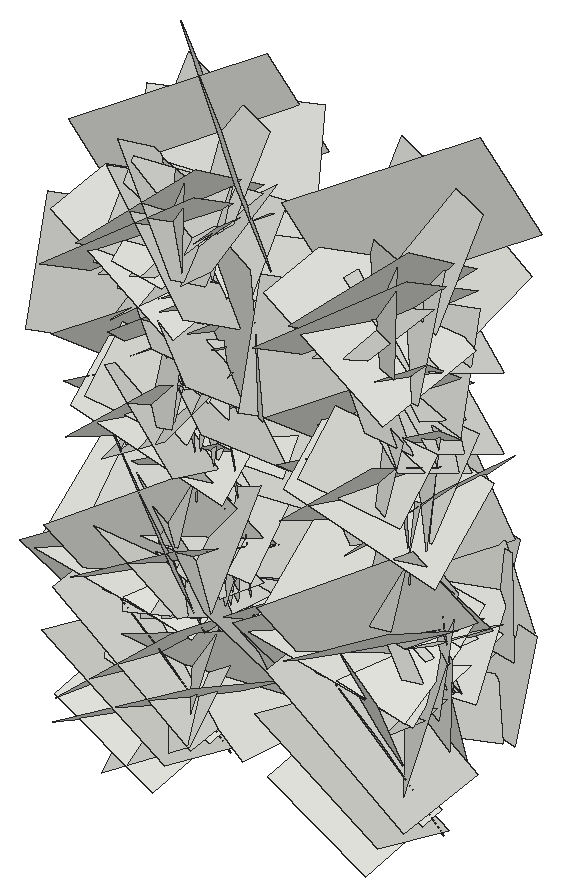
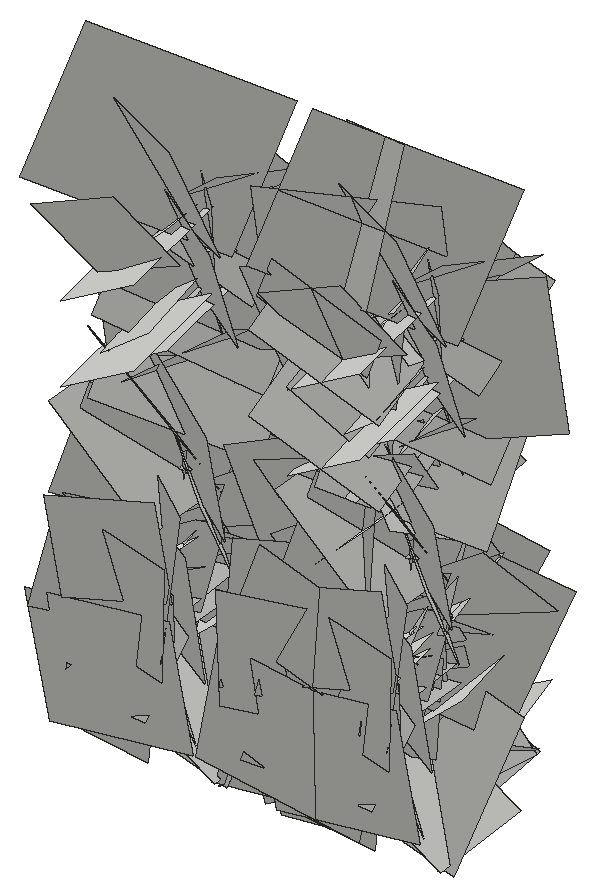
# SketchUp Ruby script. Lengths in inches.
U = 1.inch
M = Sketchup.active_model
def pt(a) = Geom::Point3d.new(a.map { |v| v * U })
def face(e, loops, mat)
  f = e.add_face(loops[0].map { |a| pt(a) })
  loops[1..].each { |l| e.add_face(l.map { |a| pt(a) }).erase! }
  f.material = f.back_material = mat if mat
  f
end
# faces: each face lists its corners as indices into pts; further lists are holes
def faces(e, pts, list, mat = nil) = list.each { |f| face(e, (f[0].is_a?(Array) ? f : [f]).map { |l| l.map { |i| pts[i] } }, mat) }
# xy, xz, yz: faces in a plane at the given z, y or x. An outline is a flat list of corners, or four numbers for a rectangle; further outlines are holes
def ring(l) = l.size == 4 ? [[l[0], l[1]], [l[2], l[1]], [l[2], l[3]], [l[0], l[3]]] : l.each_slice(2).to_a
def flat(e, list, mat, &to3) = list.each { |f| face(e, (f[0].is_a?(Array) ? f : [f]).map { |l| ring(l).map { |u, v| to3.(u, v) } }, mat) }
def xy(e, z, list, mat = nil) = flat(e, list, mat) { |x, y| [x, y, z] }
def xz(e, y, list, mat = nil) = flat(e, list, mat) { |x, z| [x, y, z] }
def yz(e, x, list, mat = nil) = flat(e, list, mat) { |y, z| [x, y, z] }
def lines(e, pts, list) = list.each { |a, b| e.add_line(pt(pts[a]), pt(pts[b])) }
# prism: a flat outline (further loops are holes) pulled along v
def prism(e, loops, v, mat = nil)
  f = face(e, loops, mat); d = Geom::Vector3d.new(v.map { |x| x * U })
  f.pushpull(f.normal.samedirection?(d) ? d.length : -d.length)
end
def box(e, o, s, mat = nil) = prism(e, [[o, [o[0] + s[0], o[1], o[2]], [o[0] + s[0], o[1] + s[1], o[2]], [o[0], o[1] + s[1], o[2]]]], [0, 0, s[2]], mat)
def at(x, y, z, deg = 0) = Geom::Transformation.translation(pt([x, y, z])) * Geom::Transformation.rotation(ORIGIN, Z_AXIS, deg.degrees)
def axes(o, x, y, z) = Geom::Transformation.new([*x, 0, *y, 0, *z, 0, *pt(o).to_a, 1])
def part(name) = M.definitions.add(name)
# library, detail: a bought-in or finely detailed component or shape, given as its bounding box
def library(name, o, s) = part(name).tap { |d| box(d.entities, o, s) }
def detail(e, o, s) = box(e.add_group.entities, o, s)
def put(e, d, t, mat = nil) = e.add_instance(d, t).tap { |i| i.material = mat if mat }
def group(e, t, mat = nil) = e.add_group.tap { |g| g.transformation = t; g.material = mat if mat }.entities
root = M.entities
c1 = part("Component\#6")
p = [[0.01,0,0],[0,3.24,4.54],[4.32,3.24,4.54],[4.33,0,0]]
faces(c1.entities,p,[[0,1,2,3]])
put(root,c1,axes([410.71,208.64,6.82],[0.0498,0.28937,-0.67344],[0.06797,-0.67386,-0.28508],[0.77398,0.04056,0.06836]))
put(root,c1,axes([404.88,210.125,0.49],[-0.19083,-0.77607,-0.35788],[-0.04853,-0.35645,0.796],[-0.90459,0.18284,0.03279]))
put(root,c1,axes([400.91,210.125,0.49],[0.19083,-0.77607,-0.35788],[0.04853,-0.35645,0.796],[0.90459,0.18284,0.03279]))
put(root,c1,axes([414.68,210.125,0.49],[-0.19083,-0.77607,-0.35788],[-0.04853,-0.35645,0.796],[-0.90459,0.18284,0.03279]))
put(root,c1,axes([404.88,210.53,-0.53],[0.13793,-1.11303,0.36033],[-0.12678,0.348,1.11812],[-1.23359,-0.16021,-0.07463]))
put(root,c1,axes([400.91,210.53,-0.53],[-0.13793,-1.11303,0.36033],[0.12678,0.348,1.11812],[1.23359,-0.16021,-0.07463]))
put(root,c1,axes([414.68,210.53,-0.53],[0.13793,-1.11303,0.36033],[-0.12678,0.348,1.11812],[-1.23359,-0.16021,-0.07463]))
put(root,c1,axes([404.88,209.89,15.21],[-0.14915,-0.31655,-0.61374],[-0.00846,-0.62556,0.32448],[-0.73195,0.07174,0.12131]))
put(root,c1,axes([400.91,209.89,15.21],[0.14915,-0.31655,-0.61374],[0.00846,-0.62556,0.32448],[0.73195,0.07174,0.12131]))
put(root,c1,axes([414.68,209.89,15.21],[-0.14915,-0.31655,-0.61374],[-0.00846,-0.62556,0.32448],[-0.73195,0.07174,0.12131]))
put(root,c1,axes([400.91,209.73,11.28],[-0.10776,-0.78869,0.28769],[-0.10217,0.29884,0.7852],[0.88401,-0.0616,0.12582]))
put(root,c1,axes([404.88,209.73,11.28],[0.10776,-0.78869,0.28769],[0.10217,0.29884,0.7852],[-0.88401,-0.0616,0.12582]))
put(root,c1,axes([410.71,209.73,11.28],[-0.10776,-0.78869,0.28769],[-0.10217,0.29884,0.7852],[0.88401,-0.0616,0.12582]))
put(root,c1,axes([404.88,208.44,11.85],[0.18719,0.63062,-0.8853],[0.07209,-0.90156,-0.62864],[-1.1499,0.04614,-0.18352]))
put(root,c1,axes([414.68,208.44,11.85],[0.18719,0.63062,-0.8853],[0.07209,-0.90156,-0.62864],[-1.1499,0.04614,-0.18352]))
put(root,c1,axes([400.91,208.44,11.85],[-0.18719,0.63062,-0.8853],[-0.07209,-0.90156,-0.62864],[1.1499,0.04614,-0.18352]))
put(root,c1,axes([404.88,206.93,9.09],[0.09893,0.82066,-0.28112],[-0.08874,-0.2729,-0.82446],[-0.91523,0.11517,0.04956]))
put(root,c1,axes([400.91,206.93,9.09],[-0.09893,0.82066,-0.28112],[0.08874,-0.2729,-0.82446],[0.91523,0.11517,0.04956]))
put(root,c1,axes([414.68,206.93,9.09],[0.09893,0.82066,-0.28112],[-0.08874,-0.2729,-0.82446],[-0.91523,0.11517,0.04956]))
put(root,c1,axes([400.91,210.2,16.34],[-0.08816,-0.12898,-0.67949],[0.09646,-0.68047,0.11803],[0.72675,0.07467,-0.09809]))
put(root,c1,axes([404.88,210.2,16.34],[0.08816,-0.12898,-0.67949],[-0.09646,-0.68047,0.11803],[-0.72675,0.07467,-0.09809]))
put(root,c1,axes([410.71,210.2,16.34],[-0.08816,-0.12898,-0.67949],[0.09646,-0.68047,0.11803],[0.72675,0.07467,-0.09809]))
put(root,c1,axes([400.91,208.78,18.92],[0.08317,0.53287,-0.42892],[-0.0846,-0.42165,-0.53844],[0.72013,-0.11108,-0.01372]))
put(root,c1,axes([404.88,208.78,18.92],[-0.08317,0.53287,-0.42892],[0.0846,-0.42165,-0.53844],[-0.72013,-0.11108,-0.01372]))
put(root,c1,axes([410.71,208.78,18.92],[0.08317,0.53287,-0.42892],[-0.0846,-0.42165,-0.53844],[0.72013,-0.11108,-0.01372]))
put(root,c1,axes([404.88,212.18,1.04],[0.25647,-1.30664,0.09966],[0.13645,0.12456,1.32049],[-1.38234,-0.23013,0.14883]))
put(root,c1,axes([400.91,212.18,1.04],[-0.25647,-1.30664,0.09966],[-0.13645,0.12456,1.32049],[1.38234,-0.23013,0.14883]))
put(root,c1,axes([414.68,212.18,1.04],[0.25647,-1.30664,0.09966],[0.13645,0.12456,1.32049],[-1.38234,-0.23013,0.14883]))
put(root,c1,axes([404.88,208.07,23.15],[-0.06368,1.0247,-0.55961],[0.10104,-0.55418,-1.02498],[-1.23347,-0.0983,-0.05507]))
put(root,c1,axes([400.91,208.07,23.15],[0.06368,1.0247,-0.55961],[-0.10104,-0.55418,-1.02498],[1.23347,-0.0983,-0.05507]))
put(root,c1,axes([414.68,208.07,23.15],[-0.06368,1.0247,-0.55961],[0.10104,-0.55418,-1.02498],[-1.23347,-0.0983,-0.05507]))
put(root,c1,axes([400.91,211.39,19.29],[-0.15412,-0.67583,-0.24542],[0.06417,-0.26101,0.68288],[0.75944,-0.11509,-0.10751]))
put(root,c1,axes([404.88,211.39,19.29],[0.15412,-0.67583,-0.24542],[-0.06417,-0.26101,0.68288],[-0.75944,-0.11509,-0.10751]))
put(root,c1,axes([410.71,211.39,19.29],[-0.15412,-0.67583,-0.24542],[0.06417,-0.26101,0.68288],[0.75944,-0.11509,-0.10751]))
put(root,c1,axes([400.91,210.2,18.35],[-0.0434,-0.8468,0.50557],[-0.21084,0.5027,0.82588],[1.02393,0.06762,0.19149]))
put(root,c1,axes([404.88,210.2,18.35],[0.0434,-0.8468,0.50557],[0.21084,0.5027,0.82588],[-1.02393,0.06762,0.19149]))
put(root,c1,axes([410.71,210.2,18.35],[-0.0434,-0.8468,0.50557],[-0.21084,0.5027,0.82588],[1.02393,0.06762,0.19149]))
put(root,c1,axes([404.88,211.18,6.7],[-0.06152,-0.66215,-0.45123],[-0.20693,-0.42709,0.65185],[-0.82377,0.15673,-0.13005]))
put(root,c1,axes([400.91,211.18,6.7],[0.06152,-0.66215,-0.45123],[0.20693,-0.42709,0.65185],[0.82377,0.15673,-0.13005]))
put(root,c1,axes([414.68,211.18,6.7],[-0.06152,-0.66215,-0.45123],[-0.20693,-0.42709,0.65185],[-0.82377,0.15673,-0.13005]))
put(root,c1,axes([404.88,209.17,10.9],[0.01303,0.87895,-0.98683],[0.04513,-0.98662,-0.87824],[-1.40007,-0.02362,-0.03749]))
put(root,c1,axes([400.91,209.17,10.9],[-0.01303,0.87895,-0.98683],[-0.04513,-0.98662,-0.87824],[1.40007,-0.02362,-0.03749]))
put(root,c1,axes([414.68,209.17,10.9],[0.01303,0.87895,-0.98683],[0.04513,-0.98662,-0.87824],[-1.40007,-0.02362,-0.03749]))
put(root,c1,axes([404.88,212.1,18.5625],[-0.14567,-1.06407,-0.312],[0.08976,-0.32354,1.06612],[-1.17197,0.10748,0.12044]))
put(root,c1,axes([400.91,212.1,18.5625],[0.14567,-1.06407,-0.312],[-0.08976,-0.32354,1.06612],[1.17197,0.10748,0.12044]))
put(root,c1,axes([414.68,212.1,18.5625],[-0.14567,-1.06407,-0.312],[0.08976,-0.32354,1.06612],[-1.17197,0.10748,0.12044]))
put(root,c1,axes([404.88,212.58,7.86],[-0.11208,-0.8157,-0.84783],[0.04176,-0.85323,0.81597],[-1.2464,0.04476,0.10358]))
put(root,c1,axes([400.91,212.58,7.86],[0.11208,-0.8157,-0.84783],[-0.04176,-0.85323,0.81597],[1.2464,0.04476,0.10358]))
put(root,c1,axes([414.68,212.58,7.86],[-0.11208,-0.8157,-0.84783],[0.04176,-0.85323,0.81597],[-1.2464,0.04476,0.10358]))
put(root,c1,axes([404.88,213.11,12.64],[0.17797,-1.01022,-0.50589],[0.14692,-0.48916,1.02282],[-1.18855,-0.21174,0.05069]))
put(root,c1,axes([400.91,213.11,12.64],[-0.17797,-1.01022,-0.50589],[-0.14692,-0.48916,1.02282],[1.18855,-0.21174,0.05069]))
put(root,c1,axes([414.68,213.11,12.64],[0.17797,-1.01022,-0.50589],[0.14692,-0.48916,1.02282],[-1.18855,-0.21174,0.05069]))
put(root,c1,axes([404.88,207.33,19.43],[-0.19308,0.28824,0.9525],[0.12727,0.96762,-0.26985],[-1.04716,0.06445,-0.20842]))
put(root,c1,axes([414.68,207.33,19.43],[-0.19308,0.28824,0.9525],[0.12727,0.96762,-0.26985],[-1.04716,0.06445,-0.20842]))
put(root,c1,axes([400.91,207.33,19.43],[0.19308,0.28824,0.9525],[-0.12727,0.96762,-0.26985],[1.04716,0.06445,-0.20842]))
put(root,c1,axes([404.88,209.23,19.24],[-0.2079,0.89177,-0.6436],[0.06754,-0.64344,-0.91097],[-1.16379,-0.19665,0.06211]))
put(root,c1,axes([400.91,209.23,19.24],[0.2079,0.89177,-0.6436],[-0.06754,-0.64344,-0.91097],[1.16379,-0.19665,0.06211]))
put(root,c1,axes([414.68,209.23,19.24],[-0.2079,0.89177,-0.6436],[0.06754,-0.64344,-0.91097],[-1.16379,-0.19665,0.06211]))
put(root,c1,axes([400.91,209.48,12.42],[0.00847,0.47556,-0.37402],[0.05873,-0.37306,-0.47315],[0.63863,0.028,0.04848]))
put(root,c1,axes([404.88,209.48,12.42],[-0.00847,0.47556,-0.37402],[-0.05873,-0.37306,-0.47315],[-0.63863,0.028,0.04848]))
put(root,c1,axes([410.71,209.48,12.42],[0.00847,0.47556,-0.37402],[0.05873,-0.37306,-0.47315],[0.63863,0.028,0.04848]))
put(root,c1,axes([404.88,207.16,9.13],[-0.13241,0.57393,0.92472],[0.131,0.93225,-0.56191],[-1.14619,0.04024,-0.17105]))
put(root,c1,axes([400.91,207.16,9.13],[0.13241,0.57393,0.92472],[-0.131,0.93225,-0.56191],[1.14619,0.04024,-0.17105]))
put(root,c1,axes([414.68,207.16,9.13],[-0.13241,0.57393,0.92472],[0.131,0.93225,-0.56191],[-1.14619,0.04024,-0.17105]))
put(root,c1,axes([404.88,212.32,20.17],[-0.18703,-0.0568,-1.36224],[-0.02248,-1.37332,0.06001],[-1.44505,0.02871,0.17537]))
put(root,c1,axes([400.91,212.32,20.17],[0.18703,-0.0568,-1.36224],[0.02248,-1.37332,0.06001],[1.44505,0.02871,0.17537]))
put(root,c1,axes([414.68,212.32,20.17],[-0.18703,-0.0568,-1.36224],[-0.02248,-1.37332,0.06001],[-1.44505,0.02871,0.17537]))
put(root,c1,axes([400.91,211.74,12.76],[0.12736,-0.0958,-0.74557],[-0.10526,-0.75044,0.08042],[0.78982,-0.08457,0.13094]))
put(root,c1,axes([404.88,211.74,12.76],[-0.12736,-0.0958,-0.74557],[0.10526,-0.75044,0.08042],[-0.78982,-0.08457,0.13094]))
put(root,c1,axes([410.71,211.74,12.76],[0.12736,-0.0958,-0.74557],[-0.10526,-0.75044,0.08042],[0.78982,-0.08457,0.13094]))
put(root,c1,axes([404.88,209.9375,16.21],[-0.25577,0.83815,-0.61941],[-0.04278,-0.64283,-0.85412],[-1.10389,-0.16928,0.17662]))
put(root,c1,axes([400.91,209.9375,16.21],[0.25577,0.83815,-0.61941],[0.04278,-0.64283,-0.85412],[1.10389,-0.16928,0.17662]))
put(root,c1,axes([414.68,209.9375,16.21],[-0.25577,0.83815,-0.61941],[-0.04278,-0.64283,-0.85412],[-1.10389,-0.16928,0.17662]))
put(root,c1,axes([404.88,210.25,-0.65],[-0.14226,-0.69765,1.16631],[-0.2044,1.1699,0.67761],[-1.42601,-0.0981,-0.21348]))
put(root,c1,axes([400.91,210.25,-0.65],[0.14226,-0.69765,1.16631],[0.2044,1.1699,0.67761],[1.42601,-0.0981,-0.21348]))
put(root,c1,axes([414.68,210.25,-0.65],[-0.14226,-0.69765,1.16631],[-0.2044,1.1699,0.67761],[-1.42601,-0.0981,-0.21348]))
put(root,c1,axes([404.88,208.82,8.26],[0.05727,0.78185,-0.16779],[-0.14528,-0.15663,-0.77398],[-0.83509,0.08087,0.12314]))
put(root,c1,axes([414.68,208.82,8.26],[0.05727,0.78185,-0.16779],[-0.14528,-0.15663,-0.77398],[-0.83509,0.08087,0.12314]))
put(root,c1,axes([400.91,208.82,8.26],[-0.05727,0.78185,-0.16779],[0.14528,-0.15663,-0.77398],[0.83509,0.08087,0.12314]))
put(root,c1,axes([404.88,211.87,13.61],[-0.09122,-0.87293,0.35057],[0.03759,0.34878,0.87716],[-0.99643,0.09307,0.001]))
put(root,c1,axes([400.91,211.87,13.61],[0.09122,-0.87293,0.35057],[-0.03759,0.34878,0.87716],[0.99643,0.09307,0.001]))
put(root,c1,axes([414.68,211.87,13.61],[-0.09122,-0.87293,0.35057],[0.03759,0.34878,0.87716],[-0.99643,0.09307,0.001]))
put(root,c1,axes([400.91,210.23,8.89],[0.07411,0.69071,-0.39914],[-0.11234,-0.38908,-0.69186],[0.83811,-0.11323,-0.05744]))
put(root,c1,axes([404.88,210.23,8.89],[-0.07411,0.69071,-0.39914],[0.11234,-0.38908,-0.69186],[-0.83811,-0.11323,-0.05744]))
put(root,c1,axes([410.71,210.23,8.89],[0.07411,0.69071,-0.39914],[-0.11234,-0.38908,-0.69186],[0.83811,-0.11323,-0.05744]))
put(root,c1,axes([404.88,208.7,17.77],[-0.06939,0.44909,1.0594],[-0.12824,1.05255,-0.45366],[-1.21294,-0.13697,-0.01265]))
put(root,c1,axes([414.68,208.7,17.77],[-0.06939,0.44909,1.0594],[-0.12824,1.05255,-0.45366],[-1.21294,-0.13697,-0.01265]))
put(root,c1,axes([400.91,208.7,17.77],[0.06939,0.44909,1.0594],[0.12824,1.05255,-0.45366],[1.21294,-0.13697,-0.01265]))
put(root,c1,axes([404.88,207.55,1.43],[0.12288,0.50669,1.25804],[0.22547,1.24021,-0.51911],[-1.41983,0.2408,0.02645]))
put(root,c1,axes([400.91,207.55,1.43],[-0.12288,0.50669,1.25804],[-0.22547,1.24021,-0.51911],[1.41983,0.2408,0.02645]))
put(root,c1,axes([414.68,207.55,1.43],[0.12288,0.50669,1.25804],[0.22547,1.24021,-0.51911],[-1.41983,0.2408,0.02645]))
put(root,c1,axes([400.91,209.4375,21.31],[-0.06259,0.84258,-0.05617],[-0.1593,-0.0659,-0.83045],[0.88082,0.04795,-0.15418]))
put(root,c1,axes([404.88,209.4375,21.31],[0.06259,0.84258,-0.05617],[0.1593,-0.0659,-0.83045],[-0.88082,0.04795,-0.15418]))
put(root,c1,axes([410.71,209.4375,21.31],[-0.06259,0.84258,-0.05617],[-0.1593,-0.0659,-0.83045],[0.88082,0.04795,-0.15418]))
put(root,c1,axes([404.88,209.66,7.46],[0.07333,0.81549,-0.13491],[-0.15326,-0.12136,-0.8077],[-0.86266,0.09088,0.13203]))
put(root,c1,axes([414.68,209.66,7.46],[0.07333,0.81549,-0.13491],[-0.15326,-0.12136,-0.8077],[-0.86266,0.09088,0.13203]))
put(root,c1,axes([400.91,209.66,7.46],[-0.07333,0.81549,-0.13491],[0.15326,-0.12136,-0.8077],[0.86266,0.09088,0.13203]))
put(root,c1,axes([400.91,208.59,6.01],[-0.08926,0.55811,0.79685],[-0.15858,0.78289,-0.56414],[1.01897,0.17073,-0.01799]))
put(root,c1,axes([404.88,208.59,6.01],[0.08926,0.55811,0.79685],[0.15858,0.78289,-0.56414],[-1.01897,0.17073,-0.01799]))
put(root,c1,axes([410.71,208.59,6.01],[-0.08926,0.55811,0.79685],[-0.15858,0.78289,-0.56414],[1.01897,0.17073,-0.01799]))
put(root,c1,axes([404.88,209.05,10.75],[-0.11444,0.37825,1.13851],[-0.07236,1.13932,-0.38499],[-1.26962,-0.09903,-0.08068]))
put(root,c1,axes([400.91,209.05,10.75],[0.11444,0.37825,1.13851],[0.07236,1.13932,-0.38499],[1.26962,-0.09903,-0.08068]))
put(root,c1,axes([414.68,209.05,10.75],[-0.11444,0.37825,1.13851],[-0.07236,1.13932,-0.38499],[-1.26962,-0.09903,-0.08068]))
put(root,c1,axes([404.88,209.13,4.61],[-0.2016,1.24111,0.06484],[0.01549,0.06782,-1.25535],[-1.31728,-0.18915,-0.02468]))
put(root,c1,axes([400.91,209.13,4.61],[0.2016,1.24111,0.06484],[-0.01549,0.06782,-1.25535],[1.31728,-0.18915,-0.02468]))
put(root,c1,axes([414.68,209.13,4.61],[-0.2016,1.24111,0.06484],[0.01549,0.06782,-1.25535],[-1.31728,-0.18915,-0.02468]))
put(root,c1,axes([400.91,210.26,8.16],[0.03239,0.64464,-0.05696],[0.08466,-0.06034,-0.64009],[0.68073,-0.02317,0.08231]))
put(root,c1,axes([404.88,210.26,8.16],[-0.03239,0.64464,-0.05696],[-0.08466,-0.06034,-0.64009],[-0.68073,-0.02317,0.08231]))
put(root,c1,axes([410.71,210.26,8.16],[0.03239,0.64464,-0.05696],[0.08466,-0.06034,-0.64009],[0.68073,-0.02317,0.08231]))
put(root,c1,axes([404.88,212.31,27.23],[0.13595,0.64817,-1.16375],[0.16935,-1.16817,-0.63303],[-1.40181,-0.07826,-0.18933]))
put(root,c1,axes([400.91,212.31,27.23],[-0.13595,0.64817,-1.16375],[-0.16935,-1.16817,-0.63303],[1.40181,-0.07826,-0.18933]))
put(root,c1,axes([414.68,212.31,27.23],[0.13595,0.64817,-1.16375],[0.16935,-1.16817,-0.63303],[-1.40181,-0.07826,-0.18933]))
put(root,c1,axes([404.88,209.54,11.71],[0.0382,0.56931,0.80625],[-0.18345,0.79793,-0.5557],[-1.03,-0.121,0.12888]))
put(root,c1,axes([400.91,209.54,11.71],[-0.0382,0.56931,0.80625],[0.18345,0.79793,-0.5557],[1.03,-0.121,0.12888]))
put(root,c1,axes([414.68,209.54,11.71],[0.0382,0.56931,0.80625],[-0.18345,0.79793,-0.5557],[-1.03,-0.121,0.12888]))
put(root,c1,axes([404.88,210.59,2.66],[0.04023,-0.02679,0.90097],[-0.06825,0.89939,0.02945],[-0.95301,-0.06554,0.03592]))
put(root,c1,axes([400.91,210.59,2.66],[-0.04023,-0.02679,0.90097],[0.06825,0.89939,0.02945],[0.95301,-0.06554,0.03592]))
put(root,c1,axes([414.68,210.59,2.66],[0.04023,-0.02679,0.90097],[-0.06825,0.89939,0.02945],[-0.95301,-0.06554,0.03592]))
put(root,c1,axes([400.91,210.86,7.98],[-0.16776,-0.30988,0.90566],[-0.16933,0.91363,0.28469],[1.00041,0.10267,0.20006]))
put(root,c1,axes([404.88,210.86,7.98],[0.16776,-0.30988,0.90566],[0.16933,0.91363,0.28469],[-1.00041,0.10267,0.20006]))
put(root,c1,axes([410.71,210.86,7.98],[-0.16776,-0.30988,0.90566],[-0.16933,0.91363,0.28469],[1.00041,0.10267,0.20006]))
put(root,c1,axes([404.88,209.9375,13.64],[0.01722,0.9911,-0.0782],[0.18047,-0.07983,-0.97637],[-1.03826,0.00256,-0.17101]))
put(root,c1,axes([400.91,209.9375,13.64],[-0.01722,0.9911,-0.0782],[-0.18047,-0.07983,-0.97637],[1.03826,0.00256,-0.17101]))
put(root,c1,axes([414.68,209.9375,13.64],[0.01722,0.9911,-0.0782],[0.18047,-0.07983,-0.97637],[-1.03826,0.00256,-0.17101]))
put(root,c1,axes([404.88,209.74,20.23],[0.19527,0.38459,1.04089],[-0.21918,1.04855,-0.35083],[-1.15564,-0.13388,0.24241]))
put(root,c1,axes([414.68,209.74,20.23],[0.19527,0.38459,1.04089],[-0.21918,1.04855,-0.35083],[-1.15564,-0.13388,0.24241]))
put(root,c1,axes([400.91,209.74,20.23],[-0.19527,0.38459,1.04089],[0.21918,1.04855,-0.35083],[1.15564,-0.13388,0.24241]))
put(root,c1,axes([404.88,209.94,4.23],[0.07499,0.16237,1.17608],[-0.09639,1.17545,-0.15681],[-1.25477,-0.08059,0.08234]))
put(root,c1,axes([400.91,209.94,4.23],[-0.07499,0.16237,1.17608],[0.09639,1.17545,-0.15681],[1.25477,-0.08059,0.08234]))
put(root,c1,axes([414.68,209.94,4.23],[0.07499,0.16237,1.17608],[-0.09639,1.17545,-0.15681],[-1.25477,-0.08059,0.08234]))
put(root,c1,axes([400.91,211.25,18.13],[0.01725,0.58763,-0.23192],[-0.06908,-0.2292,-0.5853],[0.66607,-0.03899,-0.0547]))
put(root,c1,axes([404.88,211.25,18.13],[-0.01725,0.58763,-0.23192],[0.06908,-0.2292,-0.5853],[-0.66607,-0.03899,-0.0547]))
put(root,c1,axes([410.71,211.25,18.13],[0.01725,0.58763,-0.23192],[-0.06908,-0.2292,-0.5853],[0.66607,-0.03899,-0.0547]))
put(root,c1,axes([404.88,210.82,6.78],[-0.05791,0.63342,0.22945],[-0.07755,0.22326,-0.63376],[-0.7099,-0.07606,0.05052]))
put(root,c1,axes([400.91,210.82,6.78],[0.05791,0.63342,0.22945],[0.07755,0.22326,-0.63376],[0.7099,-0.07606,0.05052]))
put(root,c1,axes([410.71,210.82,6.78],[0.05791,0.63342,0.22945],[0.07755,0.22326,-0.63376],[0.7099,-0.07606,0.05052]))
put(root,c1,axes([404.88,213.68,13.61],[-0.09122,-0.87293,0.35057],[0.03759,0.34878,0.87716],[-0.99643,0.09307,0.001]))
put(root,c1,axes([404.88,213.68,16.94],[-0.09122,-0.87293,0.35057],[0.03759,0.34878,0.87716],[-0.99643,0.09307,0.001]))
put(root,c1,axes([400.91,213.68,13.61],[0.09122,-0.87293,0.35057],[-0.03759,0.34878,0.87716],[0.99643,0.09307,0.001]))
put(root,c1,axes([400.91,213.68,16.94],[0.09122,-0.87293,0.35057],[-0.03759,0.34878,0.87716],[0.99643,0.09307,0.001]))
put(root,c1,axes([414.68,213.68,13.61],[-0.09122,-0.87293,0.35057],[0.03759,0.34878,0.87716],[-0.99643,0.09307,0.001]))
put(root,c1,axes([414.68,213.68,16.94],[-0.09122,-0.87293,0.35057],[0.03759,0.34878,0.87716],[-0.99643,0.09307,0.001]))
put(root,c1,axes([404.88,210.81,4.97],[-0.03332,-0.20638,1.23099],[0.11506,1.22627,0.20836],[-1.31805,0.11226,-0.01293]))
put(root,c1,axes([400.91,210.81,4.97],[0.03332,-0.20638,1.23099],[-0.11506,1.22627,0.20836],[1.31805,0.11226,-0.01293]))
put(root,c1,axes([414.68,210.81,4.97],[-0.03332,-0.20638,1.23099],[0.11506,1.22627,0.20836],[-1.31805,0.11226,-0.01293]))
put(root,c1,axes([400.91,213.28,4.19],[0.08194,0.11028,-0.62172],[0.07302,-0.6241,-0.10214],[0.66532,0.05491,0.08778]))
put(root,c1,axes([404.88,213.28,4.19],[-0.08194,0.11028,-0.62172],[-0.07302,-0.6241,-0.10214],[-0.66532,0.05491,0.08778]))
put(root,c1,axes([410.71,213.28,4.19],[0.08194,0.11028,-0.62172],[0.07302,-0.6241,-0.10214],[0.66532,0.05491,0.08778]))
put(root,c1,axes([400.91,211.49,4.24],[-0.12406,-0.24562,0.96087],[-0.14629,0.96216,0.22914],[1.04104,0.10594,0.1467]))
put(root,c1,axes([404.88,211.49,4.24],[0.12406,-0.24562,0.96087],[0.14629,0.96216,0.22914],[-1.04104,0.10594,0.1467]))
put(root,c1,axes([410.71,211.49,4.24],[-0.12406,-0.24562,0.96087],[-0.14629,0.96216,0.22914],[1.04104,0.10594,0.1467]))
put(root,c1,axes([404.88,213.625,2.08],[-0.05814,-0.55559,0.66869],[-0.23916,0.65616,0.52668],[-0.88998,-0.14003,-0.18522]))
put(root,c1,axes([400.91,213.625,2.08],[0.05814,-0.55559,0.66869],[0.23916,0.65616,0.52668],[0.88998,-0.14003,-0.18522]))
put(root,c1,axes([414.68,213.625,2.08],[-0.05814,-0.55559,0.66869],[-0.23916,0.65616,0.52668],[-0.88998,-0.14003,-0.18522]))
put(root,c1,axes([405.56,214.43,20.82],[-0.40689,-0.33066,-0.61889],[-0.38957,-0.50621,0.4984],[-0.63361,0.52358,0.09101]))
put(root,c1,axes([400.23,214.43,20.82],[0.40689,-0.33066,-0.61889],[0.38957,-0.50621,0.4984],[0.63361,0.52358,0.09101]))
put(root,c1,axes([415.36,214.43,20.82],[-0.40689,-0.33066,-0.61889],[-0.38957,-0.50621,0.4984],[-0.63361,0.52358,0.09101]))
put(root,c1,axes([400.34,214.33,3.125],[0.1239,-0.08914,-0.58356],[0.39991,-0.44626,0.14373],[0.48128,0.39377,0.0308]))
put(root,c1,axes([405.45,214.33,3.125],[-0.1239,-0.08914,-0.58356],[-0.39991,-0.44626,0.14373],[-0.48128,0.39377,0.0308]))
put(root,c1,axes([410.14,214.33,3.125],[0.1239,-0.08914,-0.58356],[0.39991,-0.44626,0.14373],[0.48128,0.39377,0.0308]))
put(root,c1,axes([405.04,213.9375,9.46],[0.03176,-0.01156,-1.03134],[-0.82675,-0.67538,-0.01509],[-0.71538,0.78001,-0.02835]))
put(root,c1,axes([400.75,213.9375,9.46],[-0.03176,-0.01156,-1.03134],[0.82675,-0.67538,-0.01509],[0.71538,0.78001,-0.02835]))
put(root,c1,axes([414.84,213.9375,9.46],[0.03176,-0.01156,-1.03134],[-0.82675,-0.67538,-0.01509],[-0.71538,0.78001,-0.02835]))
put(root,c1,axes([400.29,214.375,11.05],[-0.24885,0.08416,-0.78609],[0.48118,-0.65702,-0.20591],[0.6861,0.4913,-0.14071]))
put(root,c1,axes([405.5,214.375,11.05],[0.24885,0.08416,-0.78609],[-0.48118,-0.65702,-0.20591],[-0.6861,0.4913,-0.14071]))
put(root,c1,axes([410.09,214.375,11.05],[-0.24885,0.08416,-0.78609],[0.48118,-0.65702,-0.20591],[0.6861,0.4913,-0.14071]))
put(root,c1,axes([405.69,214.56,5.98],[-0.23258,-0.01173,-1.12749],[-0.77314,-0.87447,0.15104],[-0.91146,0.74476,0.15959]))
put(root,c1,axes([400.1,214.56,5.98],[0.23258,-0.01173,-1.12749],[0.77314,-0.87447,0.15104],[0.91146,0.74476,0.15959]))
put(root,c1,axes([415.5,214.56,5.98],[-0.23258,-0.01173,-1.12749],[-0.77314,-0.87447,0.15104],[-0.91146,0.74476,0.15959]))
